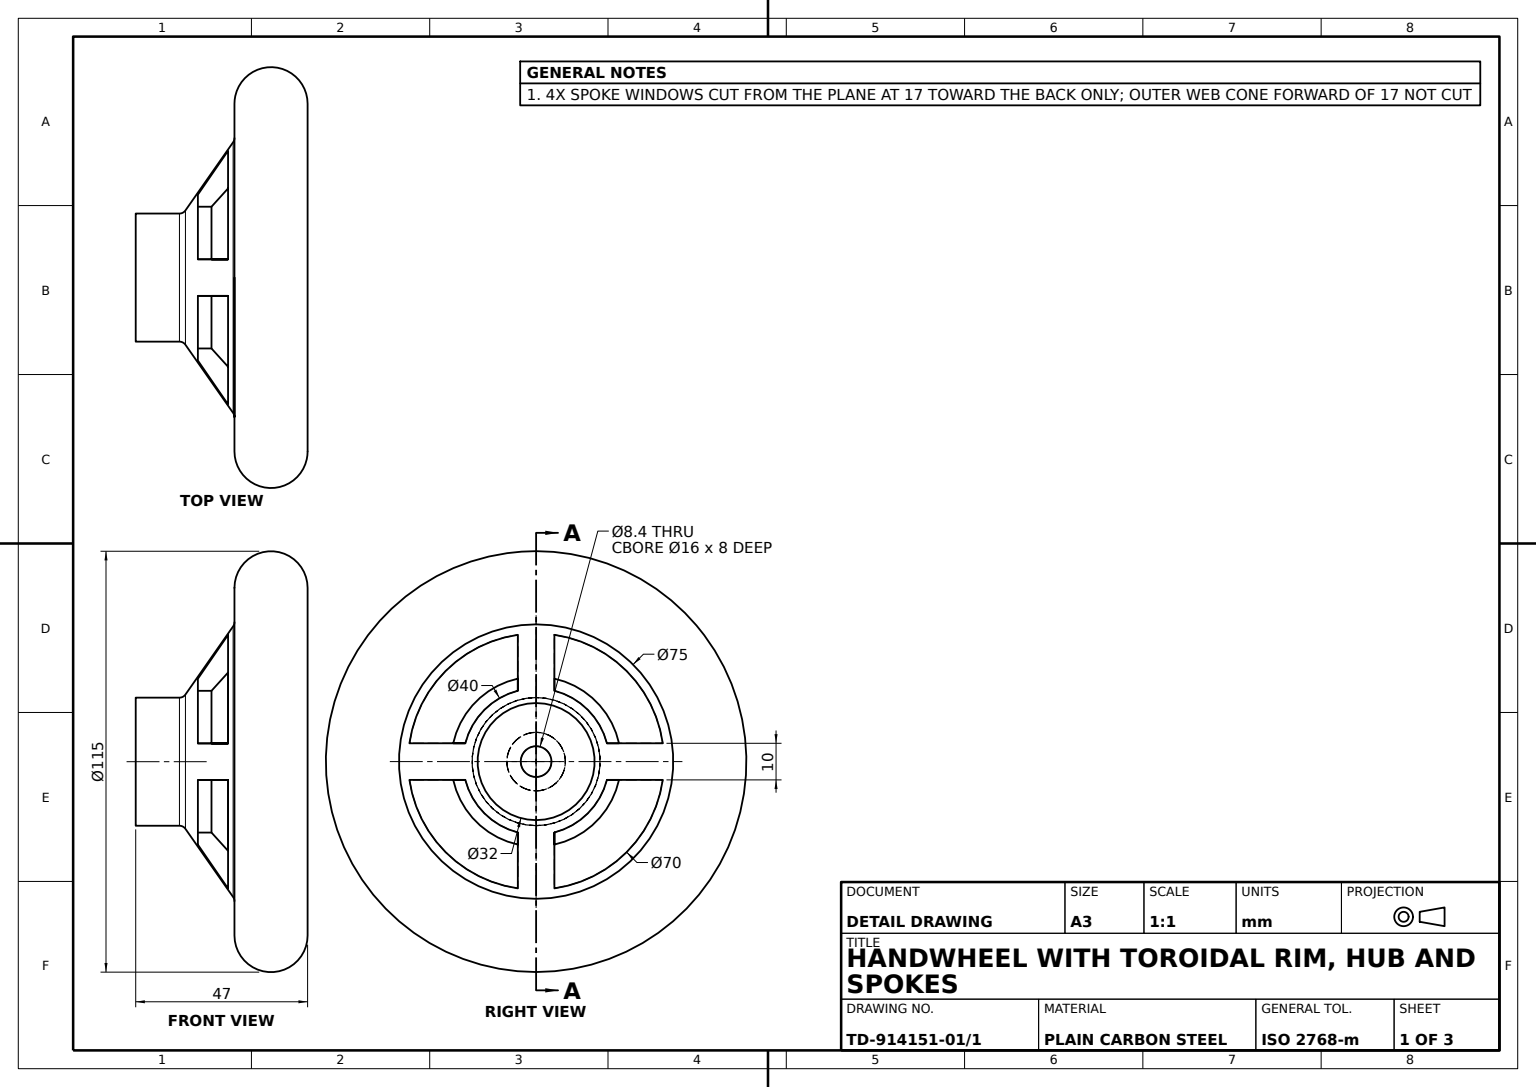
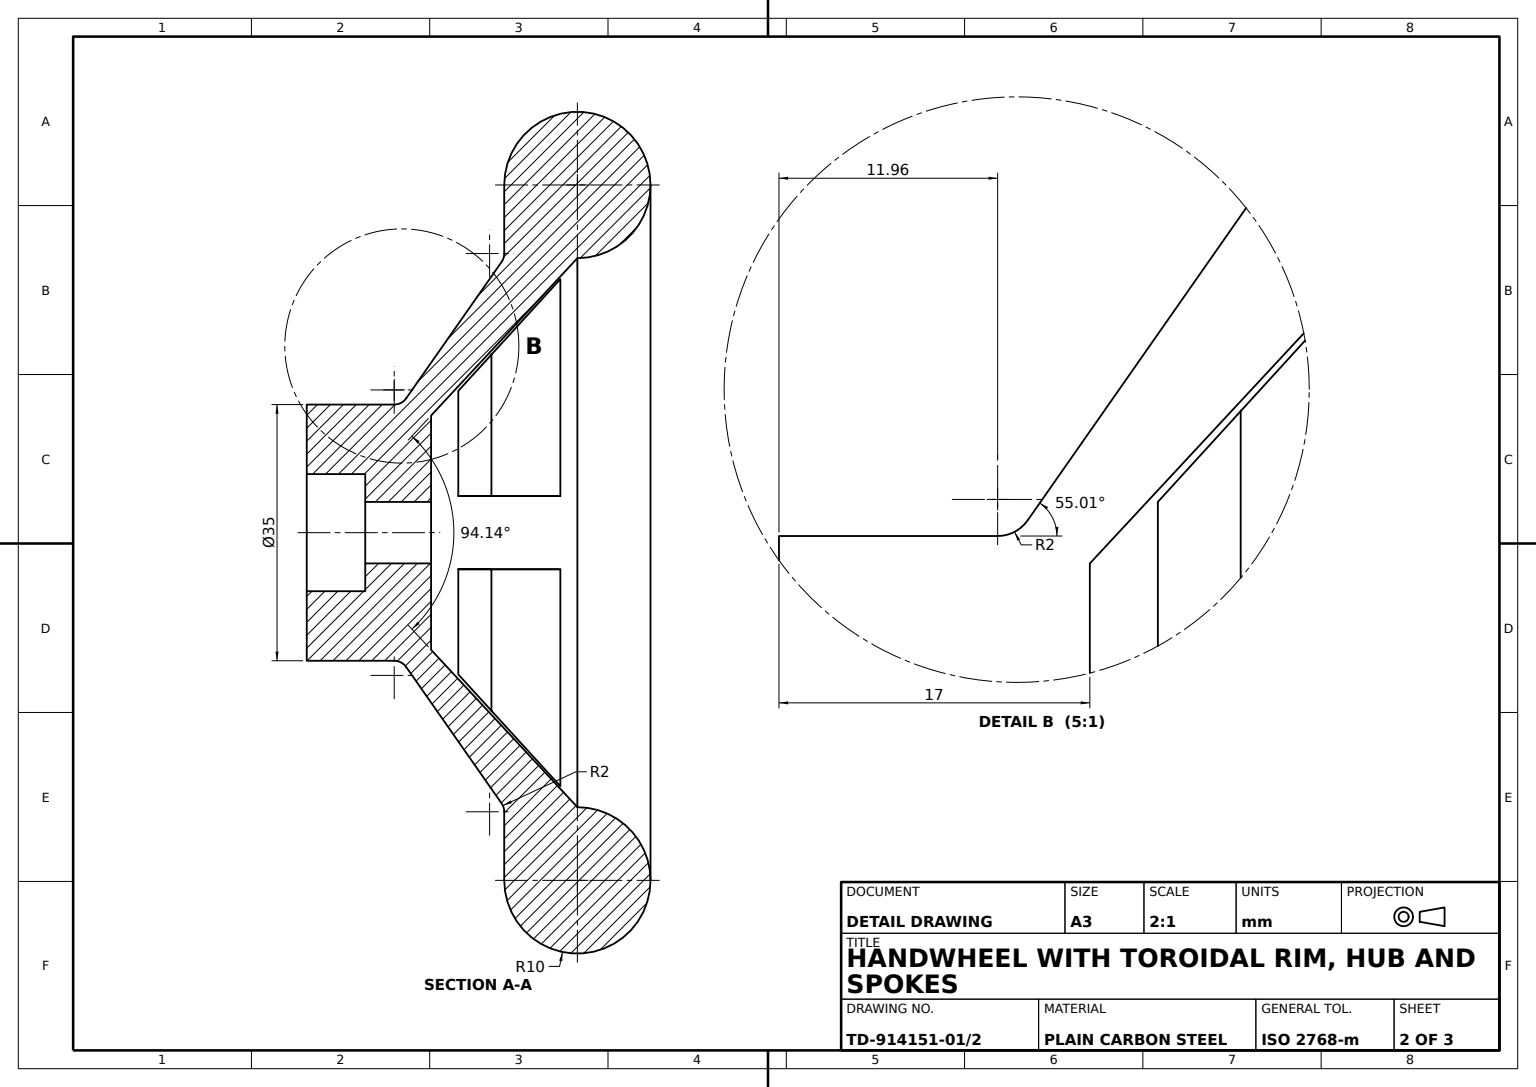
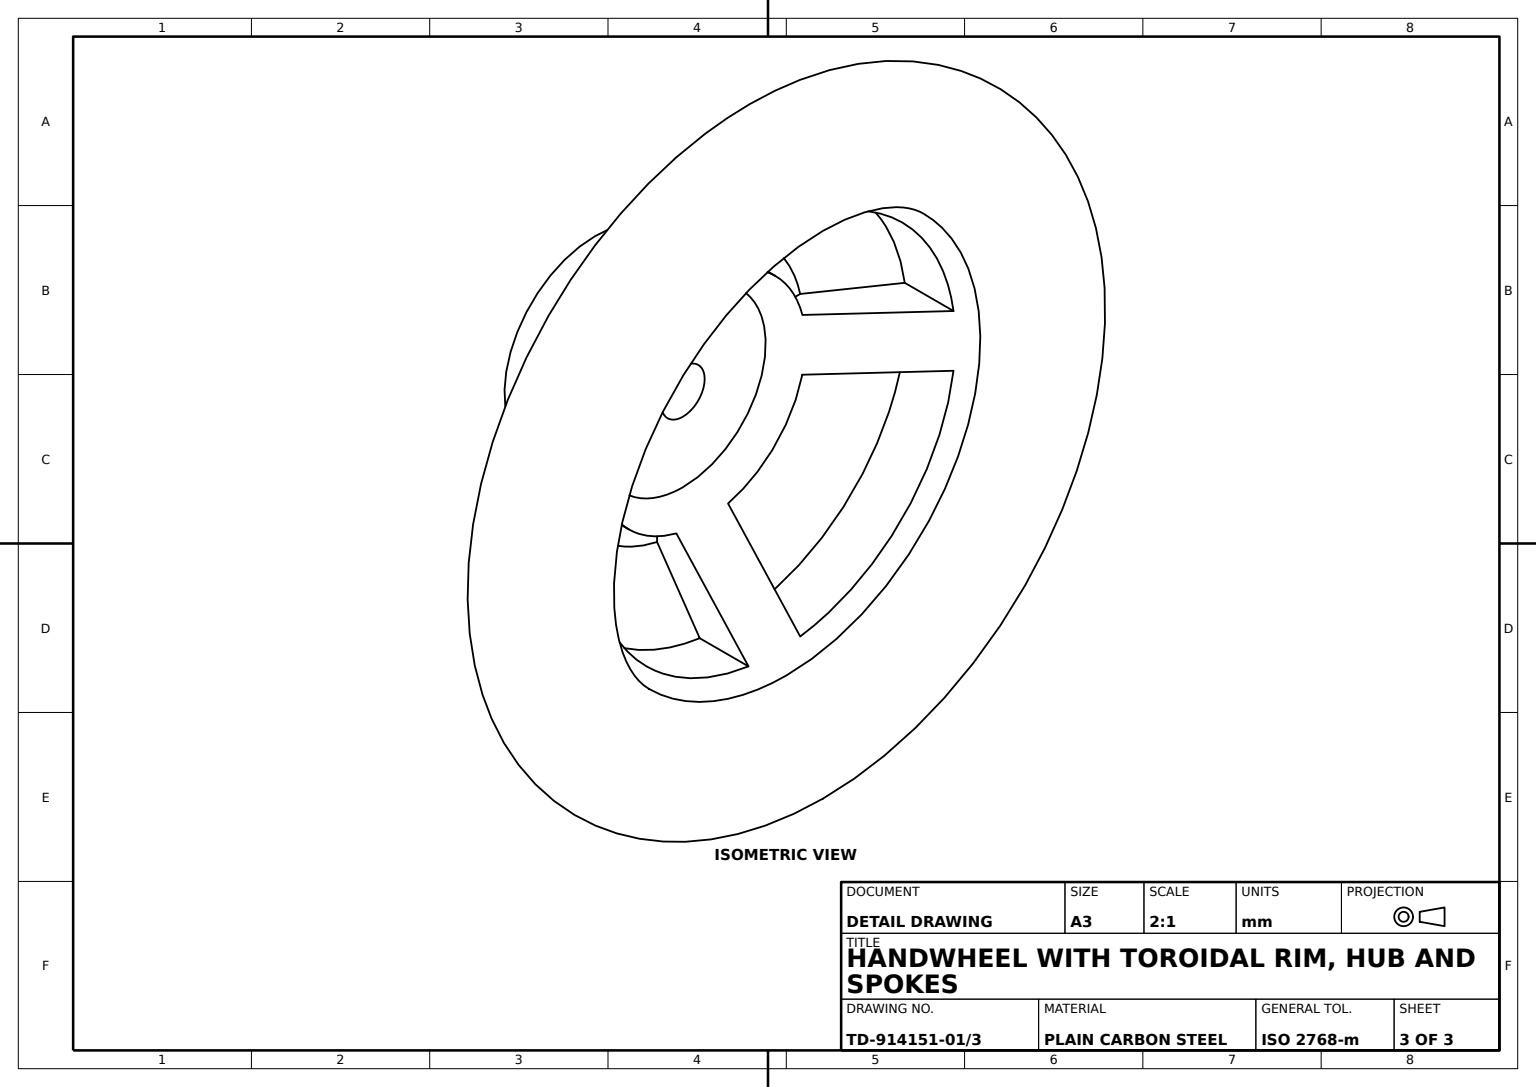
ISO-10303-21;
HEADER;
FILE_DESCRIPTION((''),'2;1');
FILE_NAME('','',(''),(''),'','','');
FILE_SCHEMA(('AUTOMOTIVE_DESIGN'));
ENDSEC;
DATA;
#1=APPLICATION_CONTEXT('');
#2=PRODUCT_CONTEXT('',#1,'mechanical');
#3=PRODUCT('','','',(#2));
#4=PRODUCT_DEFINITION_FORMATION('','',#3);
#5=PRODUCT_DEFINITION_CONTEXT('',#1,'design');
#6=PRODUCT_DEFINITION('','',#4,#5);
#7=PRODUCT_DEFINITION_SHAPE('','',#6);
#8=(LENGTH_UNIT()NAMED_UNIT(*)SI_UNIT(.MILLI.,.METRE.));
#9=(NAMED_UNIT(*)PLANE_ANGLE_UNIT()SI_UNIT($,.RADIAN.));
#10=(NAMED_UNIT(*)SI_UNIT($,.STERADIAN.)SOLID_ANGLE_UNIT());
#11=UNCERTAINTY_MEASURE_WITH_UNIT(LENGTH_MEASURE(1.E-05),#8,'distance_accuracy_value','');
#12=(GEOMETRIC_REPRESENTATION_CONTEXT(3)GLOBAL_UNCERTAINTY_ASSIGNED_CONTEXT((#11))GLOBAL_UNIT_ASSIGNED_CONTEXT((#8,#9,#10))REPRESENTATION_CONTEXT('',''));
#13=CARTESIAN_POINT('',(5.,-16.27907,-19.364917));
#14=VERTEX_POINT('',#13);
#15=CARTESIAN_POINT('',(5.,-20.,-19.364917));
#16=VERTEX_POINT('',#15);
#17=CARTESIAN_POINT('',(5.,0.,-19.364917));
#18=DIRECTION('',(0.,-1.,0.));
#19=VECTOR('',#18,1000.);
#20=LINE('',#17,#19);
#21=EDGE_CURVE('',#14,#16,#20,.T.);
#22=ORIENTED_EDGE('',*,*,#21,.T.);
#23=CARTESIAN_POINT('',(5.,-20.,-22.66943));
#24=VERTEX_POINT('',#23);
#25=CARTESIAN_POINT('',(5.,-20.,0.));
#26=DIRECTION('',(0.,0.,1.));
#27=VECTOR('',#26,1000.);
#28=LINE('',#25,#27);
#29=EDGE_CURVE('',#24,#16,#28,.T.);
#30=ORIENTED_EDGE('',*,*,#29,.F.);
#31=CARTESIAN_POINT('',(5.,-11.75,-34.641016));
#32=VERTEX_POINT('',#31);
#33=CARTESIAN_POINT('',(5.,-14.509969,-30.657344));
#34=CARTESIAN_POINT('',(5.,-17.265095,-26.670341));
#35=B_SPLINE_CURVE_WITH_KNOTS('',3,(#31,#33,#34,#23),.UNSPECIFIED.,.F.,.F.,(4,4),(0.021999232,0.036538187),.UNSPECIFIED.);
#36=EDGE_CURVE('',#32,#24,#35,.T.);
#37=ORIENTED_EDGE('',*,*,#36,.F.);
#38=CARTESIAN_POINT('',(5.,-2.325581,-34.641016));
#39=VERTEX_POINT('',#38);
#40=CARTESIAN_POINT('',(5.,0.,-34.641016));
#41=LINE('',#40,#19);
#42=EDGE_CURVE('',#39,#32,#41,.T.);
#43=ORIENTED_EDGE('',*,*,#42,.F.);
#44=CARTESIAN_POINT('',(5.,-13.971393,-21.927027));
#45=CARTESIAN_POINT('',(5.,-11.649112,-24.476011));
#46=CARTESIAN_POINT('',(5.,-6.99436,-29.564818));
#47=CARTESIAN_POINT('',(5.,-4.661293,-32.104106));
#48=B_SPLINE_CURVE_WITH_KNOTS('',3,(#13,#44,#45,#46,#47,#38),.UNSPECIFIED.,.F.,.F.,(4,2,4),(0.030560526,0.040917085,0.051273643),.UNSPECIFIED.);
#49=EDGE_CURVE('',#14,#39,#48,.T.);
#50=ORIENTED_EDGE('',*,*,#49,.F.);
#51=EDGE_LOOP('',(#22,#30,#37,#43,#50));
#52=FACE_OUTER_BOUND('',#51,.T.);
#53=CARTESIAN_POINT('',(5.,0.,0.));
#54=DIRECTION('',(1.,0.,0.));
#55=DIRECTION('',(0.,1.,0.));
#56=AXIS2_PLACEMENT_3D('',#53,#54,#55);
#57=PLANE('',#56);
#58=ADVANCED_FACE('',(#52),#57,.T.);
#59=CARTESIAN_POINT('',(-4.2,-29.,0.));
#60=VERTEX_POINT('',#59);
#61=CARTESIAN_POINT('',(-4.2,-20.,0.));
#62=VERTEX_POINT('',#61);
#63=CARTESIAN_POINT('',(-4.2,48.530716,0.));
#64=VECTOR('',#55,1000.);
#65=LINE('',#63,#64);
#66=EDGE_CURVE('',#60,#62,#65,.T.);
#67=ORIENTED_EDGE('',*,*,#66,.F.);
#68=CARTESIAN_POINT('',(4.2,-29.,0.));
#69=VERTEX_POINT('',#68);
#70=CARTESIAN_POINT('',(0.,-29.,0.));
#71=DIRECTION('',(-1.,0.,0.));
#72=AXIS2_PLACEMENT_3D('',#70,#55,#71);
#73=CIRCLE('',#72,4.2);
#74=EDGE_CURVE('',#69,#60,#73,.T.);
#75=ORIENTED_EDGE('',*,*,#74,.F.);
#76=CARTESIAN_POINT('',(4.2,-20.,0.));
#77=VERTEX_POINT('',#76);
#78=CARTESIAN_POINT('',(4.2,48.530716,0.));
#79=LINE('',#78,#64);
#80=EDGE_CURVE('',#69,#77,#79,.T.);
#81=ORIENTED_EDGE('',*,*,#80,.T.);
#82=CARTESIAN_POINT('',(0.,-20.,0.));
#83=AXIS2_PLACEMENT_3D('',#82,#55,#71);
#84=CIRCLE('',#83,4.2);
#85=EDGE_CURVE('',#77,#62,#84,.T.);
#86=ORIENTED_EDGE('',*,*,#85,.T.);
#87=EDGE_LOOP('',(#67,#75,#81,#86));
#88=FACE_OUTER_BOUND('',#87,.T.);
#89=CARTESIAN_POINT('',(0.,48.530716,0.));
#90=AXIS2_PLACEMENT_3D('',#89,#55,#71);
#91=CYLINDRICAL_SURFACE('',#90,4.2);
#92=ADVANCED_FACE('',(#88),#91,.F.);
#93=CARTESIAN_POINT('',(-37.5,0.,0.));
#94=VERTEX_POINT('',#93);
#95=CARTESIAN_POINT('',(37.5,0.,0.));
#96=VERTEX_POINT('',#95);
#97=CARTESIAN_POINT('',(0.,0.,0.));
#98=AXIS2_PLACEMENT_3D('',#97,#55,#71);
#99=CIRCLE('',#98,37.5);
#100=EDGE_CURVE('',#94,#96,#99,.T.);
#101=ORIENTED_EDGE('',*,*,#100,.F.);
#102=CARTESIAN_POINT('',(-47.5,-10.,0.));
#103=VERTEX_POINT('',#102);
#104=CARTESIAN_POINT('',(-47.5,0.,0.));
#105=DIRECTION('',(0.,0.,-1.));
#106=AXIS2_PLACEMENT_3D('',#104,#105,#71);
#107=CIRCLE('',#106,10.);
#108=EDGE_CURVE('',#103,#94,#107,.T.);
#109=ORIENTED_EDGE('',*,*,#108,.F.);
#110=CARTESIAN_POINT('',(47.5,-10.,0.));
#111=VERTEX_POINT('',#110);
#112=CARTESIAN_POINT('',(0.,-10.,0.));
#113=AXIS2_PLACEMENT_3D('',#112,#55,#71);
#114=CIRCLE('',#113,47.5);
#115=EDGE_CURVE('',#103,#111,#114,.T.);
#116=ORIENTED_EDGE('',*,*,#115,.T.);
#117=CARTESIAN_POINT('',(47.5,0.,0.));
#118=AXIS2_PLACEMENT_3D('',#117,#26,#54);
#119=CIRCLE('',#118,10.);
#120=EDGE_CURVE('',#111,#96,#119,.T.);
#121=ORIENTED_EDGE('',*,*,#120,.T.);
#122=EDGE_LOOP('',(#101,#109,#116,#121));
#123=FACE_OUTER_BOUND('',#122,.T.);
#124=TOROIDAL_SURFACE('',#98,47.5,10.);
#125=ADVANCED_FACE('',(#123),#124,.T.);
#126=CARTESIAN_POINT('',(5.,-20.,19.364917));
#127=VERTEX_POINT('',#126);
#128=CARTESIAN_POINT('',(19.364917,-20.,5.));
#129=VERTEX_POINT('',#128);
#130=CIRCLE('',#83,20.);
#131=EDGE_CURVE('',#127,#129,#130,.T.);
#132=ORIENTED_EDGE('',*,*,#131,.F.);
#133=CARTESIAN_POINT('',(5.,-20.,22.66943));
#134=VERTEX_POINT('',#133);
#135=EDGE_CURVE('',#127,#134,#28,.T.);
#136=ORIENTED_EDGE('',*,*,#135,.T.);
#137=CARTESIAN_POINT('',(22.66943,-20.,5.));
#138=VERTEX_POINT('',#137);
#139=AXIS2_PLACEMENT_3D('',#82,#18,#71);
#140=CIRCLE('',#139,23.214286);
#141=EDGE_CURVE('',#138,#134,#140,.T.);
#142=ORIENTED_EDGE('',*,*,#141,.F.);
#143=CARTESIAN_POINT('',(0.,-20.,5.));
#144=VECTOR('',#54,1000.);
#145=LINE('',#143,#144);
#146=EDGE_CURVE('',#129,#138,#145,.T.);
#147=ORIENTED_EDGE('',*,*,#146,.F.);
#148=EDGE_LOOP('',(#132,#136,#142,#147));
#149=FACE_OUTER_BOUND('',#148,.T.);
#150=PLANE('',#83);
#151=ADVANCED_FACE('',(#149),#150,.T.);
#152=CARTESIAN_POINT('',(-22.66943,-20.,-5.));
#153=VERTEX_POINT('',#152);
#154=CARTESIAN_POINT('',(-5.,-20.,-22.66943));
#155=VERTEX_POINT('',#154);
#156=EDGE_CURVE('',#153,#155,#140,.T.);
#157=ORIENTED_EDGE('',*,*,#156,.F.);
#158=CARTESIAN_POINT('',(-19.364917,-20.,-5.));
#159=VERTEX_POINT('',#158);
#160=CARTESIAN_POINT('',(-34.641016,-20.,-5.));
#161=LINE('',#160,#144);
#162=EDGE_CURVE('',#153,#159,#161,.T.);
#163=ORIENTED_EDGE('',*,*,#162,.T.);
#164=CARTESIAN_POINT('',(-5.,-20.,-19.364917));
#165=VERTEX_POINT('',#164);
#166=EDGE_CURVE('',#165,#159,#130,.T.);
#167=ORIENTED_EDGE('',*,*,#166,.F.);
#168=CARTESIAN_POINT('',(-5.,-20.,-34.641016));
#169=LINE('',#168,#27);
#170=EDGE_CURVE('',#155,#165,#169,.T.);
#171=ORIENTED_EDGE('',*,*,#170,.F.);
#172=EDGE_LOOP('',(#157,#163,#167,#171));
#173=FACE_OUTER_BOUND('',#172,.T.);
#174=ADVANCED_FACE('',(#173),#150,.T.);
#175=ORIENTED_EDGE('',*,*,#21,.F.);
#176=CARTESIAN_POINT('',(19.364917,-16.27907,-5.));
#177=VERTEX_POINT('',#176);
#178=CARTESIAN_POINT('',(0.,-16.27907,0.));
#179=AXIS2_PLACEMENT_3D('',#178,#18,#71);
#180=CIRCLE('',#179,20.);
#181=EDGE_CURVE('',#14,#177,#180,.T.);
#182=ORIENTED_EDGE('',*,*,#181,.T.);
#183=CARTESIAN_POINT('',(19.364917,-20.,-5.));
#184=VERTEX_POINT('',#183);
#185=CARTESIAN_POINT('',(19.364917,0.,-5.));
#186=LINE('',#185,#19);
#187=EDGE_CURVE('',#177,#184,#186,.T.);
#188=ORIENTED_EDGE('',*,*,#187,.T.);
#189=EDGE_CURVE('',#184,#16,#130,.T.);
#190=ORIENTED_EDGE('',*,*,#189,.T.);
#191=EDGE_LOOP('',(#175,#182,#188,#190));
#192=FACE_OUTER_BOUND('',#191,.T.);
#193=AXIS2_PLACEMENT_3D('',#97,#18,#54);
#194=CYLINDRICAL_SURFACE('',#193,20.);
#195=ADVANCED_FACE('',(#192),#194,.T.);
#196=ORIENTED_EDGE('',*,*,#156,.T.);
#197=CARTESIAN_POINT('',(-5.,-11.75,-34.641016));
#198=VERTEX_POINT('',#197);
#199=CARTESIAN_POINT('',(-5.,-14.509969,-30.657344));
#200=CARTESIAN_POINT('',(-5.,-17.265095,-26.670341));
#201=B_SPLINE_CURVE_WITH_KNOTS('',3,(#197,#199,#200,#154),.UNSPECIFIED.,.F.,.F.,(4,4),(0.021999232,0.036538187),.UNSPECIFIED.);
#202=EDGE_CURVE('',#198,#155,#201,.T.);
#203=ORIENTED_EDGE('',*,*,#202,.F.);
#204=CARTESIAN_POINT('',(-34.641016,-11.75,-5.));
#205=VERTEX_POINT('',#204);
#206=CARTESIAN_POINT('',(0.,-11.75,0.));
#207=AXIS2_PLACEMENT_3D('',#206,#55,#71);
#208=CIRCLE('',#207,35.);
#209=EDGE_CURVE('',#198,#205,#208,.T.);
#210=ORIENTED_EDGE('',*,*,#209,.T.);
#211=CARTESIAN_POINT('',(-30.657344,-14.509969,-5.));
#212=CARTESIAN_POINT('',(-26.670341,-17.265095,-5.));
#213=B_SPLINE_CURVE_WITH_KNOTS('',3,(#204,#211,#212,#152),.UNSPECIFIED.,.F.,.F.,(4,4),(0.021999232,0.036538187),.UNSPECIFIED.);
#214=EDGE_CURVE('',#205,#153,#213,.T.);
#215=ORIENTED_EDGE('',*,*,#214,.T.);
#216=EDGE_LOOP('',(#196,#203,#210,#215));
#217=FACE_BOUND('',#216,.T.);
#218=ORIENTED_EDGE('',*,*,#36,.T.);
#219=CARTESIAN_POINT('',(22.66943,-20.,-5.));
#220=VERTEX_POINT('',#219);
#221=EDGE_CURVE('',#24,#220,#140,.T.);
#222=ORIENTED_EDGE('',*,*,#221,.T.);
#223=CARTESIAN_POINT('',(34.641016,-11.75,-5.));
#224=VERTEX_POINT('',#223);
#225=CARTESIAN_POINT('',(26.670386,-17.265065,-5.));
#226=CARTESIAN_POINT('',(30.657374,-14.509949,-5.));
#227=B_SPLINE_CURVE_WITH_KNOTS('',3,(#219,#225,#226,#223),.UNSPECIFIED.,.F.,.F.,(4,4),(0.024878675,0.039392675),.UNSPECIFIED.);
#228=EDGE_CURVE('',#220,#224,#227,.T.);
#229=ORIENTED_EDGE('',*,*,#228,.T.);
#230=EDGE_CURVE('',#224,#32,#208,.T.);
#231=ORIENTED_EDGE('',*,*,#230,.T.);
#232=EDGE_LOOP('',(#218,#222,#229,#231));
#233=FACE_BOUND('',#232,.T.);
#234=CARTESIAN_POINT('',(18.353075,-23.402847,0.));
#235=VERTEX_POINT('',#234);
#236=CARTESIAN_POINT('',(36.98352,-10.361536,0.));
#237=VERTEX_POINT('',#236);
#238=DIRECTION('',(0.819231921,0.573462344,0.));
#239=VECTOR('',#238,1000.);
#240=LINE('',#236,#239);
#241=EDGE_CURVE('',#235,#237,#240,.T.);
#242=ORIENTED_EDGE('',*,*,#241,.F.);
#243=CARTESIAN_POINT('',(-18.353075,-23.402847,0.));
#244=VERTEX_POINT('',#243);
#245=CARTESIAN_POINT('',(0.,-23.402847,0.));
#246=AXIS2_PLACEMENT_3D('',#245,#55,#71);
#247=CIRCLE('',#246,18.353075);
#248=EDGE_CURVE('',#235,#244,#247,.T.);
#249=ORIENTED_EDGE('',*,*,#248,.T.);
#250=CARTESIAN_POINT('',(-36.98352,-10.361536,0.));
#251=VERTEX_POINT('',#250);
#252=DIRECTION('',(-0.819231921,0.573462344,0.));
#253=VECTOR('',#252,1000.);
#254=LINE('',#250,#253);
#255=EDGE_CURVE('',#244,#251,#254,.T.);
#256=ORIENTED_EDGE('',*,*,#255,.T.);
#257=CARTESIAN_POINT('',(0.,-10.361536,0.));
#258=AXIS2_PLACEMENT_3D('',#257,#55,#71);
#259=CIRCLE('',#258,36.98352);
#260=EDGE_CURVE('',#237,#251,#259,.T.);
#261=ORIENTED_EDGE('',*,*,#260,.F.);
#262=EDGE_LOOP('',(#242,#249,#256,#261));
#263=FACE_OUTER_BOUND('',#262,.T.);
#264=CONICAL_SURFACE('',#258,36.983519773,0.960070362);
#265=ADVANCED_FACE('',(#217,#233,#263),#264,.T.);
#266=EDGE_CURVE('',#60,#69,#73,.T.);
#267=ORIENTED_EDGE('',*,*,#266,.T.);
#268=ORIENTED_EDGE('',*,*,#74,.T.);
#269=EDGE_LOOP('',(#267,#268));
#270=FACE_BOUND('',#269,.T.);
#271=CARTESIAN_POINT('',(-8.,-29.,0.));
#272=VERTEX_POINT('',#271);
#273=CARTESIAN_POINT('',(8.,-29.,0.));
#274=VERTEX_POINT('',#273);
#275=CIRCLE('',#72,8.);
#276=EDGE_CURVE('',#272,#274,#275,.T.);
#277=ORIENTED_EDGE('',*,*,#276,.F.);
#278=EDGE_CURVE('',#274,#272,#275,.T.);
#279=ORIENTED_EDGE('',*,*,#278,.F.);
#280=EDGE_LOOP('',(#277,#279));
#281=FACE_OUTER_BOUND('',#280,.T.);
#282=AXIS2_PLACEMENT_3D('',#59,#18,#54);
#283=PLANE('',#282);
#284=ADVANCED_FACE('',(#270,#281),#283,.T.);
#285=CARTESIAN_POINT('',(-19.364917,-16.27907,5.));
#286=VERTEX_POINT('',#285);
#287=CARTESIAN_POINT('',(-34.641016,-2.325581,5.));
#288=VERTEX_POINT('',#287);
#289=CARTESIAN_POINT('',(-21.927027,-13.971393,5.));
#290=CARTESIAN_POINT('',(-24.476011,-11.649112,5.));
#291=CARTESIAN_POINT('',(-29.564818,-6.99436,5.));
#292=CARTESIAN_POINT('',(-32.104106,-4.661293,5.));
#293=B_SPLINE_CURVE_WITH_KNOTS('',3,(#285,#289,#290,#291,#292,#287),.UNSPECIFIED.,.F.,.F.,(4,2,4),(0.030560526,0.040917085,0.051273643),.UNSPECIFIED.);
#294=EDGE_CURVE('',#286,#288,#293,.T.);
#295=ORIENTED_EDGE('',*,*,#294,.T.);
#296=CARTESIAN_POINT('',(-34.641016,-11.75,5.));
#297=VERTEX_POINT('',#296);
#298=CARTESIAN_POINT('',(-34.641016,0.,5.));
#299=LINE('',#298,#19);
#300=EDGE_CURVE('',#288,#297,#299,.T.);
#301=ORIENTED_EDGE('',*,*,#300,.T.);
#302=CARTESIAN_POINT('',(-22.66943,-20.,5.));
#303=VERTEX_POINT('',#302);
#304=CARTESIAN_POINT('',(-30.657344,-14.509969,5.));
#305=CARTESIAN_POINT('',(-26.670341,-17.265095,5.));
#306=B_SPLINE_CURVE_WITH_KNOTS('',3,(#296,#304,#305,#302),.UNSPECIFIED.,.F.,.F.,(4,4),(0.021999232,0.036538187),.UNSPECIFIED.);
#307=EDGE_CURVE('',#297,#303,#306,.T.);
#308=ORIENTED_EDGE('',*,*,#307,.T.);
#309=CARTESIAN_POINT('',(-19.364917,-20.,5.));
#310=VERTEX_POINT('',#309);
#311=CARTESIAN_POINT('',(-34.641016,-20.,5.));
#312=LINE('',#311,#144);
#313=EDGE_CURVE('',#303,#310,#312,.T.);
#314=ORIENTED_EDGE('',*,*,#313,.T.);
#315=CARTESIAN_POINT('',(-19.364917,0.,5.));
#316=LINE('',#315,#19);
#317=EDGE_CURVE('',#286,#310,#316,.T.);
#318=ORIENTED_EDGE('',*,*,#317,.F.);
#319=EDGE_LOOP('',(#295,#301,#308,#314,#318));
#320=FACE_OUTER_BOUND('',#319,.T.);
#321=AXIS2_PLACEMENT_3D('',#298,#105,#71);
#322=PLANE('',#321);
#323=ADVANCED_FACE('',(#320),#322,.F.);
#324=ORIENTED_EDGE('',*,*,#300,.F.);
#325=CARTESIAN_POINT('',(-5.,-2.325581,34.641016));
#326=VERTEX_POINT('',#325);
#327=CARTESIAN_POINT('',(0.,-2.325581,0.));
#328=AXIS2_PLACEMENT_3D('',#327,#18,#71);
#329=CIRCLE('',#328,35.);
#330=EDGE_CURVE('',#326,#288,#329,.T.);
#331=ORIENTED_EDGE('',*,*,#330,.F.);
#332=CARTESIAN_POINT('',(-5.,-11.75,34.641016));
#333=VERTEX_POINT('',#332);
#334=CARTESIAN_POINT('',(-5.,0.,34.641016));
#335=LINE('',#334,#19);
#336=EDGE_CURVE('',#326,#333,#335,.T.);
#337=ORIENTED_EDGE('',*,*,#336,.T.);
#338=EDGE_CURVE('',#297,#333,#208,.T.);
#339=ORIENTED_EDGE('',*,*,#338,.F.);
#340=EDGE_LOOP('',(#324,#331,#337,#339));
#341=FACE_OUTER_BOUND('',#340,.T.);
#342=CYLINDRICAL_SURFACE('',#193,35.);
#343=ADVANCED_FACE('',(#341),#342,.F.);
#344=EDGE_CURVE('',#251,#237,#259,.T.);
#345=ORIENTED_EDGE('',*,*,#344,.T.);
#346=CARTESIAN_POINT('',(38.130444,-10.,0.));
#347=VERTEX_POINT('',#346);
#348=CARTESIAN_POINT('',(38.130444,-12.,0.));
#349=AXIS2_PLACEMENT_3D('',#348,#26,#54);
#350=CIRCLE('',#349,2.);
#351=EDGE_CURVE('',#347,#237,#350,.T.);
#352=ORIENTED_EDGE('',*,*,#351,.F.);
#353=CARTESIAN_POINT('',(-38.130444,-10.,0.));
#354=VERTEX_POINT('',#353);
#355=CIRCLE('',#113,38.130444);
#356=EDGE_CURVE('',#354,#347,#355,.T.);
#357=ORIENTED_EDGE('',*,*,#356,.F.);
#358=CARTESIAN_POINT('',(-38.130444,-12.,0.));
#359=AXIS2_PLACEMENT_3D('',#358,#105,#71);
#360=CIRCLE('',#359,2.);
#361=EDGE_CURVE('',#354,#251,#360,.T.);
#362=ORIENTED_EDGE('',*,*,#361,.T.);
#363=EDGE_LOOP('',(#345,#352,#357,#362));
#364=FACE_OUTER_BOUND('',#363,.T.);
#365=CARTESIAN_POINT('',(0.,-12.,0.));
#366=AXIS2_PLACEMENT_3D('',#365,#55,#71);
#367=TOROIDAL_SURFACE('',#366,38.130444,2.);
#368=ADVANCED_FACE('',(#364),#367,.F.);
#369=ORIENTED_EDGE('',*,*,#189,.F.);
#370=CARTESIAN_POINT('',(0.,-20.,-5.));
#371=LINE('',#370,#144);
#372=EDGE_CURVE('',#184,#220,#371,.T.);
#373=ORIENTED_EDGE('',*,*,#372,.T.);
#374=ORIENTED_EDGE('',*,*,#221,.F.);
#375=ORIENTED_EDGE('',*,*,#29,.T.);
#376=EDGE_LOOP('',(#369,#373,#374,#375));
#377=FACE_OUTER_BOUND('',#376,.T.);
#378=ADVANCED_FACE('',(#377),#150,.T.);
#379=ORIENTED_EDGE('',*,*,#135,.F.);
#380=CARTESIAN_POINT('',(5.,-16.27907,19.364917));
#381=VERTEX_POINT('',#380);
#382=CARTESIAN_POINT('',(5.,0.,19.364917));
#383=LINE('',#382,#19);
#384=EDGE_CURVE('',#381,#127,#383,.T.);
#385=ORIENTED_EDGE('',*,*,#384,.F.);
#386=CARTESIAN_POINT('',(5.,-2.325581,34.641016));
#387=VERTEX_POINT('',#386);
#388=CARTESIAN_POINT('',(5.,-4.66124,32.104164));
#389=CARTESIAN_POINT('',(5.,-6.994268,29.564919));
#390=CARTESIAN_POINT('',(5.,-11.649001,24.476133));
#391=CARTESIAN_POINT('',(5.,-13.971299,21.927131));
#392=B_SPLINE_CURVE_WITH_KNOTS('',3,(#386,#388,#389,#390,#391,#380),.UNSPECIFIED.,.F.,.F.,(4,2,4),(0.034275864,0.044620633,0.054965402),.UNSPECIFIED.);
#393=EDGE_CURVE('',#387,#381,#392,.T.);
#394=ORIENTED_EDGE('',*,*,#393,.F.);
#395=CARTESIAN_POINT('',(5.,-11.75,34.641016));
#396=VERTEX_POINT('',#395);
#397=CARTESIAN_POINT('',(5.,0.,34.641016));
#398=LINE('',#397,#19);
#399=EDGE_CURVE('',#387,#396,#398,.T.);
#400=ORIENTED_EDGE('',*,*,#399,.T.);
#401=CARTESIAN_POINT('',(5.,-17.265065,26.670386));
#402=CARTESIAN_POINT('',(5.,-14.509949,30.657374));
#403=B_SPLINE_CURVE_WITH_KNOTS('',3,(#133,#401,#402,#395),.UNSPECIFIED.,.F.,.F.,(4,4),(0.024878675,0.039392675),.UNSPECIFIED.);
#404=EDGE_CURVE('',#134,#396,#403,.T.);
#405=ORIENTED_EDGE('',*,*,#404,.F.);
#406=EDGE_LOOP('',(#379,#385,#394,#400,#405));
#407=FACE_OUTER_BOUND('',#406,.T.);
#408=ADVANCED_FACE('',(#407),#57,.T.);
#409=CARTESIAN_POINT('',(-19.364917,-16.27907,-5.));
#410=VERTEX_POINT('',#409);
#411=CARTESIAN_POINT('',(-19.364917,0.,-5.));
#412=LINE('',#411,#19);
#413=EDGE_CURVE('',#410,#159,#412,.T.);
#414=ORIENTED_EDGE('',*,*,#413,.F.);
#415=CARTESIAN_POINT('',(-5.,-16.27907,-19.364917));
#416=VERTEX_POINT('',#415);
#417=EDGE_CURVE('',#410,#416,#180,.T.);
#418=ORIENTED_EDGE('',*,*,#417,.T.);
#419=CARTESIAN_POINT('',(-5.,0.,-19.364917));
#420=LINE('',#419,#19);
#421=EDGE_CURVE('',#416,#165,#420,.T.);
#422=ORIENTED_EDGE('',*,*,#421,.T.);
#423=ORIENTED_EDGE('',*,*,#166,.T.);
#424=EDGE_LOOP('',(#414,#418,#422,#423));
#425=FACE_OUTER_BOUND('',#424,.T.);
#426=ADVANCED_FACE('',(#425),#194,.T.);
#427=ORIENTED_EDGE('',*,*,#248,.F.);
#428=CARTESIAN_POINT('',(17.5,-25.041311,0.));
#429=VERTEX_POINT('',#428);
#430=CARTESIAN_POINT('',(19.5,-25.041311,0.));
#431=AXIS2_PLACEMENT_3D('',#430,#26,#54);
#432=CIRCLE('',#431,2.);
#433=EDGE_CURVE('',#235,#429,#432,.T.);
#434=ORIENTED_EDGE('',*,*,#433,.T.);
#435=CARTESIAN_POINT('',(-17.5,-25.041311,0.));
#436=VERTEX_POINT('',#435);
#437=CARTESIAN_POINT('',(0.,-25.041311,0.));
#438=AXIS2_PLACEMENT_3D('',#437,#55,#71);
#439=CIRCLE('',#438,17.5);
#440=EDGE_CURVE('',#429,#436,#439,.T.);
#441=ORIENTED_EDGE('',*,*,#440,.T.);
#442=CARTESIAN_POINT('',(-19.5,-25.041311,0.));
#443=AXIS2_PLACEMENT_3D('',#442,#105,#71);
#444=CIRCLE('',#443,2.);
#445=EDGE_CURVE('',#244,#436,#444,.T.);
#446=ORIENTED_EDGE('',*,*,#445,.F.);
#447=EDGE_LOOP('',(#427,#434,#441,#446));
#448=FACE_OUTER_BOUND('',#447,.T.);
#449=TOROIDAL_SURFACE('',#438,19.5,2.);
#450=ADVANCED_FACE('',(#448),#449,.F.);
#451=CARTESIAN_POINT('',(34.641016,-2.325581,-5.));
#452=VERTEX_POINT('',#451);
#453=CARTESIAN_POINT('',(32.104164,-4.66124,-5.));
#454=CARTESIAN_POINT('',(29.564919,-6.994268,-5.));
#455=CARTESIAN_POINT('',(24.476133,-11.649001,-5.));
#456=CARTESIAN_POINT('',(21.927131,-13.971299,-5.));
#457=B_SPLINE_CURVE_WITH_KNOTS('',3,(#451,#453,#454,#455,#456,#176),.UNSPECIFIED.,.F.,.F.,(4,2,4),(0.034275864,0.044620633,0.054965402),.UNSPECIFIED.);
#458=EDGE_CURVE('',#452,#177,#457,.T.);
#459=ORIENTED_EDGE('',*,*,#458,.F.);
#460=CARTESIAN_POINT('',(34.641016,0.,-5.));
#461=LINE('',#460,#19);
#462=EDGE_CURVE('',#452,#224,#461,.T.);
#463=ORIENTED_EDGE('',*,*,#462,.T.);
#464=ORIENTED_EDGE('',*,*,#228,.F.);
#465=ORIENTED_EDGE('',*,*,#372,.F.);
#466=ORIENTED_EDGE('',*,*,#187,.F.);
#467=EDGE_LOOP('',(#459,#463,#464,#465,#466));
#468=FACE_OUTER_BOUND('',#467,.T.);
#469=CARTESIAN_POINT('',(0.,0.,-5.));
#470=AXIS2_PLACEMENT_3D('',#469,#105,#71);
#471=PLANE('',#470);
#472=ADVANCED_FACE('',(#468),#471,.T.);
#473=CARTESIAN_POINT('',(34.641016,-2.325581,5.));
#474=VERTEX_POINT('',#473);
#475=CARTESIAN_POINT('',(19.364917,-16.27907,5.));
#476=VERTEX_POINT('',#475);
#477=CARTESIAN_POINT('',(32.104164,-4.66124,5.));
#478=CARTESIAN_POINT('',(29.564919,-6.994268,5.));
#479=CARTESIAN_POINT('',(24.476133,-11.649001,5.));
#480=CARTESIAN_POINT('',(21.927131,-13.971299,5.));
#481=B_SPLINE_CURVE_WITH_KNOTS('',3,(#473,#477,#478,#479,#480,#475),.UNSPECIFIED.,.F.,.F.,(4,2,4),(0.034275864,0.044620633,0.054965402),.UNSPECIFIED.);
#482=EDGE_CURVE('',#474,#476,#481,.T.);
#483=ORIENTED_EDGE('',*,*,#482,.F.);
#484=EDGE_CURVE('',#474,#387,#329,.T.);
#485=ORIENTED_EDGE('',*,*,#484,.T.);
#486=ORIENTED_EDGE('',*,*,#393,.T.);
#487=EDGE_CURVE('',#476,#381,#180,.T.);
#488=ORIENTED_EDGE('',*,*,#487,.F.);
#489=EDGE_LOOP('',(#483,#485,#486,#488));
#490=FACE_BOUND('',#489,.T.);
#491=CARTESIAN_POINT('',(-16.,-20.,0.));
#492=VERTEX_POINT('',#491);
#493=DIRECTION('',(-0.732186738,0.681103942,0.));
#494=VECTOR('',#493,1000.);
#495=LINE('',#491,#494);
#496=EDGE_CURVE('',#492,#94,#495,.T.);
#497=ORIENTED_EDGE('',*,*,#496,.T.);
#498=ORIENTED_EDGE('',*,*,#100,.T.);
#499=CARTESIAN_POINT('',(16.,-20.,0.));
#500=VERTEX_POINT('',#499);
#501=DIRECTION('',(0.732186738,0.681103942,0.));
#502=VECTOR('',#501,1000.);
#503=LINE('',#499,#502);
#504=EDGE_CURVE('',#500,#96,#503,.T.);
#505=ORIENTED_EDGE('',*,*,#504,.F.);
#506=CIRCLE('',#83,16.);
#507=EDGE_CURVE('',#492,#500,#506,.T.);
#508=ORIENTED_EDGE('',*,*,#507,.F.);
#509=EDGE_LOOP('',(#497,#498,#505,#508));
#510=FACE_OUTER_BOUND('',#509,.T.);
#511=CARTESIAN_POINT('',(-5.,-16.27907,19.364917));
#512=VERTEX_POINT('',#511);
#513=EDGE_CURVE('',#512,#286,#180,.T.);
#514=ORIENTED_EDGE('',*,*,#513,.F.);
#515=CARTESIAN_POINT('',(-5.,-4.66124,32.104164));
#516=CARTESIAN_POINT('',(-5.,-6.994268,29.564919));
#517=CARTESIAN_POINT('',(-5.,-11.649001,24.476133));
#518=CARTESIAN_POINT('',(-5.,-13.971299,21.927131));
#519=B_SPLINE_CURVE_WITH_KNOTS('',3,(#325,#515,#516,#517,#518,#511),.UNSPECIFIED.,.F.,.F.,(4,2,4),(0.034275864,0.044620633,0.054965402),.UNSPECIFIED.);
#520=EDGE_CURVE('',#326,#512,#519,.T.);
#521=ORIENTED_EDGE('',*,*,#520,.F.);
#522=ORIENTED_EDGE('',*,*,#330,.T.);
#523=ORIENTED_EDGE('',*,*,#294,.F.);
#524=EDGE_LOOP('',(#514,#521,#522,#523));
#525=FACE_BOUND('',#524,.T.);
#526=CONICAL_SURFACE('',#83,16.,0.821527014);
#527=ADVANCED_FACE('',(#490,#510,#525),#526,.F.);
#528=ORIENTED_EDGE('',*,*,#260,.T.);
#529=ORIENTED_EDGE('',*,*,#361,.F.);
#530=EDGE_CURVE('',#347,#354,#355,.T.);
#531=ORIENTED_EDGE('',*,*,#530,.F.);
#532=ORIENTED_EDGE('',*,*,#351,.T.);
#533=EDGE_LOOP('',(#528,#529,#531,#532));
#534=FACE_OUTER_BOUND('',#533,.T.);
#535=ADVANCED_FACE('',(#534),#367,.F.);
#536=CARTESIAN_POINT('',(17.5,-37.,0.));
#537=VERTEX_POINT('',#536);
#538=CARTESIAN_POINT('',(-17.5,-37.,0.));
#539=VERTEX_POINT('',#538);
#540=CARTESIAN_POINT('',(0.,-37.,0.));
#541=AXIS2_PLACEMENT_3D('',#540,#55,#71);
#542=CIRCLE('',#541,17.5);
#543=EDGE_CURVE('',#537,#539,#542,.T.);
#544=ORIENTED_EDGE('',*,*,#543,.F.);
#545=EDGE_CURVE('',#539,#537,#542,.T.);
#546=ORIENTED_EDGE('',*,*,#545,.F.);
#547=EDGE_LOOP('',(#544,#546));
#548=FACE_OUTER_BOUND('',#547,.T.);
#549=CARTESIAN_POINT('',(-8.,-37.,0.));
#550=VERTEX_POINT('',#549);
#551=CARTESIAN_POINT('',(8.,-37.,0.));
#552=VERTEX_POINT('',#551);
#553=CIRCLE('',#541,8.);
#554=EDGE_CURVE('',#550,#552,#553,.T.);
#555=ORIENTED_EDGE('',*,*,#554,.T.);
#556=EDGE_CURVE('',#552,#550,#553,.T.);
#557=ORIENTED_EDGE('',*,*,#556,.T.);
#558=EDGE_LOOP('',(#555,#557));
#559=FACE_BOUND('',#558,.T.);
#560=AXIS2_PLACEMENT_3D('',#549,#18,#54);
#561=PLANE('',#560);
#562=ADVANCED_FACE('',(#548,#559),#561,.T.);
#563=ORIENTED_EDGE('',*,*,#440,.F.);
#564=CARTESIAN_POINT('',(17.5,48.530716,0.));
#565=LINE('',#564,#64);
#566=EDGE_CURVE('',#537,#429,#565,.T.);
#567=ORIENTED_EDGE('',*,*,#566,.F.);
#568=ORIENTED_EDGE('',*,*,#543,.T.);
#569=CARTESIAN_POINT('',(-17.5,48.530716,0.));
#570=LINE('',#569,#64);
#571=EDGE_CURVE('',#539,#436,#570,.T.);
#572=ORIENTED_EDGE('',*,*,#571,.T.);
#573=EDGE_LOOP('',(#563,#567,#568,#572));
#574=FACE_OUTER_BOUND('',#573,.T.);
#575=CYLINDRICAL_SURFACE('',#90,17.5);
#576=ADVANCED_FACE('',(#574),#575,.T.);
#577=ORIENTED_EDGE('',*,*,#230,.F.);
#578=ORIENTED_EDGE('',*,*,#462,.F.);
#579=EDGE_CURVE('',#39,#452,#329,.T.);
#580=ORIENTED_EDGE('',*,*,#579,.F.);
#581=ORIENTED_EDGE('',*,*,#42,.T.);
#582=EDGE_LOOP('',(#577,#578,#580,#581));
#583=FACE_OUTER_BOUND('',#582,.T.);
#584=ADVANCED_FACE('',(#583),#342,.F.);
#585=ORIENTED_EDGE('',*,*,#384,.T.);
#586=ORIENTED_EDGE('',*,*,#131,.T.);
#587=CARTESIAN_POINT('',(19.364917,0.,5.));
#588=LINE('',#587,#19);
#589=EDGE_CURVE('',#476,#129,#588,.T.);
#590=ORIENTED_EDGE('',*,*,#589,.F.);
#591=ORIENTED_EDGE('',*,*,#487,.T.);
#592=EDGE_LOOP('',(#585,#586,#590,#591));
#593=FACE_OUTER_BOUND('',#592,.T.);
#594=ADVANCED_FACE('',(#593),#194,.T.);
#595=ORIENTED_EDGE('',*,*,#507,.T.);
#596=EDGE_CURVE('',#500,#492,#506,.T.);
#597=ORIENTED_EDGE('',*,*,#596,.T.);
#598=EDGE_LOOP('',(#595,#597));
#599=FACE_OUTER_BOUND('',#598,.T.);
#600=EDGE_CURVE('',#62,#77,#84,.T.);
#601=ORIENTED_EDGE('',*,*,#600,.F.);
#602=ORIENTED_EDGE('',*,*,#85,.F.);
#603=EDGE_LOOP('',(#601,#602));
#604=FACE_BOUND('',#603,.T.);
#605=AXIS2_PLACEMENT_3D('',#61,#55,#71);
#606=PLANE('',#605);
#607=ADVANCED_FACE('',(#599,#604),#606,.T.);
#608=CARTESIAN_POINT('',(34.641016,-11.75,5.));
#609=VERTEX_POINT('',#608);
#610=EDGE_CURVE('',#396,#609,#208,.T.);
#611=ORIENTED_EDGE('',*,*,#610,.F.);
#612=ORIENTED_EDGE('',*,*,#399,.F.);
#613=ORIENTED_EDGE('',*,*,#484,.F.);
#614=CARTESIAN_POINT('',(34.641016,0.,5.));
#615=LINE('',#614,#19);
#616=EDGE_CURVE('',#474,#609,#615,.T.);
#617=ORIENTED_EDGE('',*,*,#616,.T.);
#618=EDGE_LOOP('',(#611,#612,#613,#617));
#619=FACE_OUTER_BOUND('',#618,.T.);
#620=ADVANCED_FACE('',(#619),#342,.F.);
#621=CARTESIAN_POINT('',(-5.,-20.,22.66943));
#622=VERTEX_POINT('',#621);
#623=CARTESIAN_POINT('',(-5.,-17.265065,26.670386));
#624=CARTESIAN_POINT('',(-5.,-14.509949,30.657374));
#625=B_SPLINE_CURVE_WITH_KNOTS('',3,(#621,#623,#624,#332),.UNSPECIFIED.,.F.,.F.,(4,4),(0.024878675,0.039392675),.UNSPECIFIED.);
#626=EDGE_CURVE('',#622,#333,#625,.T.);
#627=ORIENTED_EDGE('',*,*,#626,.T.);
#628=ORIENTED_EDGE('',*,*,#336,.F.);
#629=ORIENTED_EDGE('',*,*,#520,.T.);
#630=CARTESIAN_POINT('',(-5.,-20.,19.364917));
#631=VERTEX_POINT('',#630);
#632=CARTESIAN_POINT('',(-5.,0.,19.364917));
#633=LINE('',#632,#19);
#634=EDGE_CURVE('',#512,#631,#633,.T.);
#635=ORIENTED_EDGE('',*,*,#634,.T.);
#636=LINE('',#630,#27);
#637=EDGE_CURVE('',#631,#622,#636,.T.);
#638=ORIENTED_EDGE('',*,*,#637,.T.);
#639=EDGE_LOOP('',(#627,#628,#629,#635,#638));
#640=FACE_OUTER_BOUND('',#639,.T.);
#641=AXIS2_PLACEMENT_3D('',#632,#54,#55);
#642=PLANE('',#641);
#643=ADVANCED_FACE('',(#640),#642,.F.);
#644=ORIENTED_EDGE('',*,*,#146,.T.);
#645=CARTESIAN_POINT('',(26.670386,-17.265065,5.));
#646=CARTESIAN_POINT('',(30.657374,-14.509949,5.));
#647=B_SPLINE_CURVE_WITH_KNOTS('',3,(#137,#645,#646,#608),.UNSPECIFIED.,.F.,.F.,(4,4),(0.024878675,0.039392675),.UNSPECIFIED.);
#648=EDGE_CURVE('',#138,#609,#647,.T.);
#649=ORIENTED_EDGE('',*,*,#648,.T.);
#650=ORIENTED_EDGE('',*,*,#616,.F.);
#651=ORIENTED_EDGE('',*,*,#482,.T.);
#652=ORIENTED_EDGE('',*,*,#589,.T.);
#653=EDGE_LOOP('',(#644,#649,#650,#651,#652));
#654=FACE_OUTER_BOUND('',#653,.T.);
#655=CARTESIAN_POINT('',(0.,0.,5.));
#656=AXIS2_PLACEMENT_3D('',#655,#105,#71);
#657=PLANE('',#656);
#658=ADVANCED_FACE('',(#654),#657,.F.);
#659=ORIENTED_EDGE('',*,*,#637,.F.);
#660=EDGE_CURVE('',#310,#631,#130,.T.);
#661=ORIENTED_EDGE('',*,*,#660,.F.);
#662=ORIENTED_EDGE('',*,*,#313,.F.);
#663=EDGE_CURVE('',#622,#303,#140,.T.);
#664=ORIENTED_EDGE('',*,*,#663,.F.);
#665=EDGE_LOOP('',(#659,#661,#662,#664));
#666=FACE_OUTER_BOUND('',#665,.T.);
#667=ADVANCED_FACE('',(#666),#150,.T.);
#668=ORIENTED_EDGE('',*,*,#496,.F.);
#669=ORIENTED_EDGE('',*,*,#596,.F.);
#670=ORIENTED_EDGE('',*,*,#504,.T.);
#671=EDGE_CURVE('',#96,#94,#99,.T.);
#672=ORIENTED_EDGE('',*,*,#671,.T.);
#673=EDGE_LOOP('',(#668,#669,#670,#672));
#674=FACE_OUTER_BOUND('',#673,.T.);
#675=ORIENTED_EDGE('',*,*,#49,.T.);
#676=ORIENTED_EDGE('',*,*,#579,.T.);
#677=ORIENTED_EDGE('',*,*,#458,.T.);
#678=ORIENTED_EDGE('',*,*,#181,.F.);
#679=EDGE_LOOP('',(#675,#676,#677,#678));
#680=FACE_BOUND('',#679,.T.);
#681=CARTESIAN_POINT('',(-5.,-2.325581,-34.641016));
#682=VERTEX_POINT('',#681);
#683=CARTESIAN_POINT('',(-5.,-13.971393,-21.927027));
#684=CARTESIAN_POINT('',(-5.,-11.649112,-24.476011));
#685=CARTESIAN_POINT('',(-5.,-6.99436,-29.564818));
#686=CARTESIAN_POINT('',(-5.,-4.661293,-32.104106));
#687=B_SPLINE_CURVE_WITH_KNOTS('',3,(#415,#683,#684,#685,#686,#681),.UNSPECIFIED.,.F.,.F.,(4,2,4),(0.030560526,0.040917085,0.051273643),.UNSPECIFIED.);
#688=EDGE_CURVE('',#416,#682,#687,.T.);
#689=ORIENTED_EDGE('',*,*,#688,.F.);
#690=ORIENTED_EDGE('',*,*,#417,.F.);
#691=CARTESIAN_POINT('',(-34.641016,-2.325581,-5.));
#692=VERTEX_POINT('',#691);
#693=CARTESIAN_POINT('',(-21.927027,-13.971393,-5.));
#694=CARTESIAN_POINT('',(-24.476011,-11.649112,-5.));
#695=CARTESIAN_POINT('',(-29.564818,-6.99436,-5.));
#696=CARTESIAN_POINT('',(-32.104106,-4.661293,-5.));
#697=B_SPLINE_CURVE_WITH_KNOTS('',3,(#409,#693,#694,#695,#696,#691),.UNSPECIFIED.,.F.,.F.,(4,2,4),(0.030560526,0.040917085,0.051273643),.UNSPECIFIED.);
#698=EDGE_CURVE('',#410,#692,#697,.T.);
#699=ORIENTED_EDGE('',*,*,#698,.T.);
#700=EDGE_CURVE('',#692,#682,#329,.T.);
#701=ORIENTED_EDGE('',*,*,#700,.T.);
#702=EDGE_LOOP('',(#689,#690,#699,#701));
#703=FACE_BOUND('',#702,.T.);
#704=ADVANCED_FACE('',(#674,#680,#703),#526,.F.);
#705=ORIENTED_EDGE('',*,*,#120,.F.);
#706=EDGE_CURVE('',#111,#103,#114,.T.);
#707=ORIENTED_EDGE('',*,*,#706,.T.);
#708=ORIENTED_EDGE('',*,*,#108,.T.);
#709=ORIENTED_EDGE('',*,*,#671,.F.);
#710=EDGE_LOOP('',(#705,#707,#708,#709));
#711=FACE_OUTER_BOUND('',#710,.T.);
#712=ADVANCED_FACE('',(#711),#124,.T.);
#713=CARTESIAN_POINT('',(-34.641016,0.,-5.));
#714=LINE('',#713,#19);
#715=EDGE_CURVE('',#692,#205,#714,.T.);
#716=ORIENTED_EDGE('',*,*,#715,.T.);
#717=ORIENTED_EDGE('',*,*,#209,.F.);
#718=CARTESIAN_POINT('',(-5.,0.,-34.641016));
#719=LINE('',#718,#19);
#720=EDGE_CURVE('',#682,#198,#719,.T.);
#721=ORIENTED_EDGE('',*,*,#720,.F.);
#722=ORIENTED_EDGE('',*,*,#700,.F.);
#723=EDGE_LOOP('',(#716,#717,#721,#722));
#724=FACE_OUTER_BOUND('',#723,.T.);
#725=ADVANCED_FACE('',(#724),#342,.F.);
#726=CARTESIAN_POINT('',(8.,48.530716,0.));
#727=LINE('',#726,#64);
#728=EDGE_CURVE('',#552,#274,#727,.T.);
#729=ORIENTED_EDGE('',*,*,#728,.T.);
#730=ORIENTED_EDGE('',*,*,#278,.T.);
#731=CARTESIAN_POINT('',(-8.,48.530716,0.));
#732=LINE('',#731,#64);
#733=EDGE_CURVE('',#550,#272,#732,.T.);
#734=ORIENTED_EDGE('',*,*,#733,.F.);
#735=ORIENTED_EDGE('',*,*,#556,.F.);
#736=EDGE_LOOP('',(#729,#730,#734,#735));
#737=FACE_OUTER_BOUND('',#736,.T.);
#738=CYLINDRICAL_SURFACE('',#90,8.);
#739=ADVANCED_FACE('',(#737),#738,.F.);
#740=ORIENTED_EDGE('',*,*,#715,.F.);
#741=ORIENTED_EDGE('',*,*,#698,.F.);
#742=ORIENTED_EDGE('',*,*,#413,.T.);
#743=ORIENTED_EDGE('',*,*,#162,.F.);
#744=ORIENTED_EDGE('',*,*,#214,.F.);
#745=EDGE_LOOP('',(#740,#741,#742,#743,#744));
#746=FACE_OUTER_BOUND('',#745,.T.);
#747=AXIS2_PLACEMENT_3D('',#713,#105,#71);
#748=PLANE('',#747);
#749=ADVANCED_FACE('',(#746),#748,.T.);
#750=ORIENTED_EDGE('',*,*,#554,.F.);
#751=ORIENTED_EDGE('',*,*,#733,.T.);
#752=ORIENTED_EDGE('',*,*,#276,.T.);
#753=ORIENTED_EDGE('',*,*,#728,.F.);
#754=EDGE_LOOP('',(#750,#751,#752,#753));
#755=FACE_OUTER_BOUND('',#754,.T.);
#756=ADVANCED_FACE('',(#755),#738,.F.);
#757=ORIENTED_EDGE('',*,*,#338,.T.);
#758=ORIENTED_EDGE('',*,*,#626,.F.);
#759=ORIENTED_EDGE('',*,*,#663,.T.);
#760=ORIENTED_EDGE('',*,*,#307,.F.);
#761=EDGE_LOOP('',(#757,#758,#759,#760));
#762=FACE_BOUND('',#761,.T.);
#763=ORIENTED_EDGE('',*,*,#141,.T.);
#764=ORIENTED_EDGE('',*,*,#404,.T.);
#765=ORIENTED_EDGE('',*,*,#610,.T.);
#766=ORIENTED_EDGE('',*,*,#648,.F.);
#767=EDGE_LOOP('',(#763,#764,#765,#766));
#768=FACE_BOUND('',#767,.T.);
#769=ORIENTED_EDGE('',*,*,#344,.F.);
#770=ORIENTED_EDGE('',*,*,#255,.F.);
#771=EDGE_CURVE('',#244,#235,#247,.T.);
#772=ORIENTED_EDGE('',*,*,#771,.T.);
#773=ORIENTED_EDGE('',*,*,#241,.T.);
#774=EDGE_LOOP('',(#769,#770,#772,#773));
#775=FACE_OUTER_BOUND('',#774,.T.);
#776=ADVANCED_FACE('',(#762,#768,#775),#264,.T.);
#777=ORIENTED_EDGE('',*,*,#688,.T.);
#778=ORIENTED_EDGE('',*,*,#720,.T.);
#779=ORIENTED_EDGE('',*,*,#202,.T.);
#780=ORIENTED_EDGE('',*,*,#170,.T.);
#781=ORIENTED_EDGE('',*,*,#421,.F.);
#782=EDGE_LOOP('',(#777,#778,#779,#780,#781));
#783=FACE_OUTER_BOUND('',#782,.T.);
#784=AXIS2_PLACEMENT_3D('',#718,#54,#55);
#785=PLANE('',#784);
#786=ADVANCED_FACE('',(#783),#785,.F.);
#787=ORIENTED_EDGE('',*,*,#600,.T.);
#788=ORIENTED_EDGE('',*,*,#80,.F.);
#789=ORIENTED_EDGE('',*,*,#266,.F.);
#790=ORIENTED_EDGE('',*,*,#66,.T.);
#791=EDGE_LOOP('',(#787,#788,#789,#790));
#792=FACE_OUTER_BOUND('',#791,.T.);
#793=ADVANCED_FACE('',(#792),#91,.F.);
#794=ORIENTED_EDGE('',*,*,#545,.T.);
#795=ORIENTED_EDGE('',*,*,#566,.T.);
#796=EDGE_CURVE('',#436,#429,#439,.T.);
#797=ORIENTED_EDGE('',*,*,#796,.F.);
#798=ORIENTED_EDGE('',*,*,#571,.F.);
#799=EDGE_LOOP('',(#794,#795,#797,#798));
#800=FACE_OUTER_BOUND('',#799,.T.);
#801=ADVANCED_FACE('',(#800),#575,.T.);
#802=ORIENTED_EDGE('',*,*,#433,.F.);
#803=ORIENTED_EDGE('',*,*,#771,.F.);
#804=ORIENTED_EDGE('',*,*,#445,.T.);
#805=ORIENTED_EDGE('',*,*,#796,.T.);
#806=EDGE_LOOP('',(#802,#803,#804,#805));
#807=FACE_OUTER_BOUND('',#806,.T.);
#808=ADVANCED_FACE('',(#807),#449,.F.);
#809=ORIENTED_EDGE('',*,*,#634,.F.);
#810=ORIENTED_EDGE('',*,*,#513,.T.);
#811=ORIENTED_EDGE('',*,*,#317,.T.);
#812=ORIENTED_EDGE('',*,*,#660,.T.);
#813=EDGE_LOOP('',(#809,#810,#811,#812));
#814=FACE_OUTER_BOUND('',#813,.T.);
#815=ADVANCED_FACE('',(#814),#194,.T.);
#816=ORIENTED_EDGE('',*,*,#356,.T.);
#817=ORIENTED_EDGE('',*,*,#530,.T.);
#818=EDGE_LOOP('',(#816,#817));
#819=FACE_BOUND('',#818,.T.);
#820=ORIENTED_EDGE('',*,*,#706,.F.);
#821=ORIENTED_EDGE('',*,*,#115,.F.);
#822=EDGE_LOOP('',(#820,#821));
#823=FACE_OUTER_BOUND('',#822,.T.);
#824=AXIS2_PLACEMENT_3D('',#102,#18,#54);
#825=PLANE('',#824);
#826=ADVANCED_FACE('',(#819,#823),#825,.T.);
#827=CLOSED_SHELL('',(#58,#92,#125,#151,#174,#195,#265,#284,#323,#343,#368,#378,#408,#426,#450,#472,#527,#535,#562,#576,#584,#594,#607,#620,#643,#658,#667,#704,#712,#725,#739,#749,#756,#776,#786,#793,#801,#808,#815,#826));
#828=MANIFOLD_SOLID_BREP('',#827);
#829=ADVANCED_BREP_SHAPE_REPRESENTATION('',(#828),#12);
#830=SHAPE_DEFINITION_REPRESENTATION(#7,#829);
ENDSEC;
END-ISO-10303-21;
